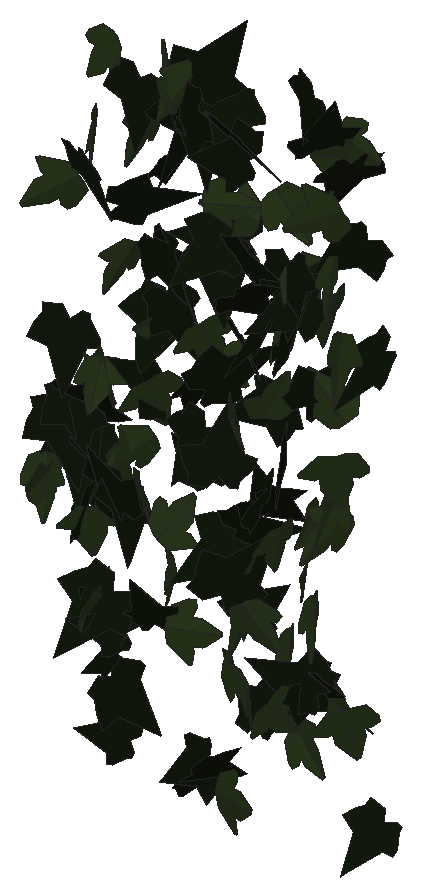
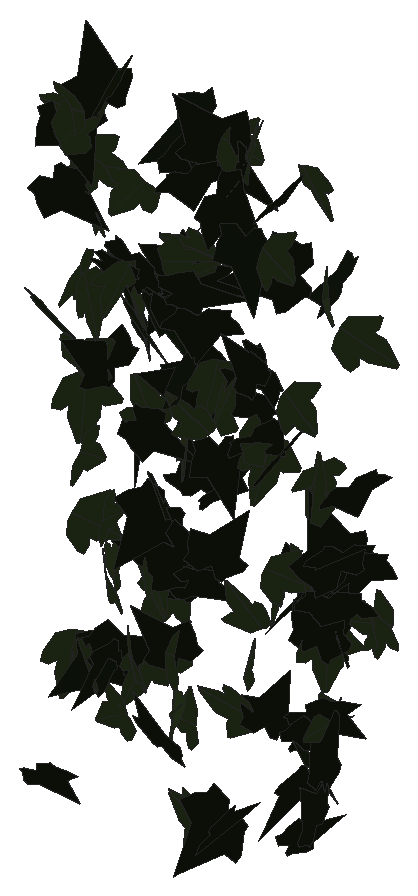
# SketchUp Ruby script. Lengths in inches.
U = 1.inch
M = Sketchup.active_model
def pt(a) = Geom::Point3d.new(a.map { |v| v * U })
def face(e, loops, mat)
  f = e.add_face(loops[0].map { |a| pt(a) })
  loops[1..].each { |l| e.add_face(l.map { |a| pt(a) }).erase! }
  f.material = f.back_material = mat if mat
  f
end
# faces: each face lists its corners as indices into pts; further lists are holes
def faces(e, pts, list, mat = nil) = list.each { |f| face(e, (f[0].is_a?(Array) ? f : [f]).map { |l| l.map { |i| pts[i] } }, mat) }
# xy, xz, yz: faces in a plane at the given z, y or x. An outline is a flat list of corners, or four numbers for a rectangle; further outlines are holes
def ring(l) = l.size == 4 ? [[l[0], l[1]], [l[2], l[1]], [l[2], l[3]], [l[0], l[3]]] : l.each_slice(2).to_a
def flat(e, list, mat, &to3) = list.each { |f| face(e, (f[0].is_a?(Array) ? f : [f]).map { |l| ring(l).map { |u, v| to3.(u, v) } }, mat) }
def xy(e, z, list, mat = nil) = flat(e, list, mat) { |x, y| [x, y, z] }
def xz(e, y, list, mat = nil) = flat(e, list, mat) { |x, z| [x, y, z] }
def yz(e, x, list, mat = nil) = flat(e, list, mat) { |y, z| [x, y, z] }
def lines(e, pts, list) = list.each { |a, b| e.add_line(pt(pts[a]), pt(pts[b])) }
# prism: a flat outline (further loops are holes) pulled along v
def prism(e, loops, v, mat = nil)
  f = face(e, loops, mat); d = Geom::Vector3d.new(v.map { |x| x * U })
  f.pushpull(f.normal.samedirection?(d) ? d.length : -d.length)
end
def box(e, o, s, mat = nil) = prism(e, [[o, [o[0] + s[0], o[1], o[2]], [o[0] + s[0], o[1] + s[1], o[2]], [o[0], o[1] + s[1], o[2]]]], [0, 0, s[2]], mat)
def at(x, y, z, deg = 0) = Geom::Transformation.translation(pt([x, y, z])) * Geom::Transformation.rotation(ORIGIN, Z_AXIS, deg.degrees)
def axes(o, x, y, z) = Geom::Transformation.new([*x, 0, *y, 0, *z, 0, *pt(o).to_a, 1])
def part(name) = M.definitions.add(name)
# library, detail: a bought-in or finely detailed component or shape, given as its bounding box
def library(name, o, s) = part(name).tap { |d| box(d.entities, o, s) }
def detail(e, o, s) = box(e.add_group.entities, o, s)
def put(e, d, t, mat = nil) = e.add_instance(d, t).tap { |i| i.material = mat if mat }
def group(e, t, mat = nil) = e.add_group.tap { |g| g.transformation = t; g.material = mat if mat }.entities
root = M.entities
M.materials.add("efeu1").color = [18, 25, 13]
M.materials.add("efeu2").color = [43, 57, 29]
c1 = part("ivyleaf_9")
p = [[1.54,2.16,1.25],[1.36,2.04,1.19],[-0.21,0.99,0.68],[-0.71,1.11,0.82],[-0.85,0.86,0.67],[-0.8,0.17,0.21],
  [-0.9,-0.01,0.1],[-0.67,-0.16,-0.02],[-0.08,-0.08,-0.05],[-0.03,-0.6,-0.4],[0.65,-0.88,-0.66],[0.83,-0.6,-0.49],
  [1.29,-0.42,-0.43],[1.8125,-0.07,-0.26],[1.21,0.44,0.15]]
faces(c1.entities,p,[[0,1,2,3,4,5,6,7,8,9,10,11,12,13,14]],"efeu1")
c2 = part("ivyleaf_10")
p = [[0,0.5,-0.03],[-0.0625,2.02,-0.43],[-0.19,2.01,-0.46],[-0.54,1.05,-0.29],[-0.52,0.625,-0.18],[-0.83,0.76,-0.28],
  [-1.16,0.64,-0.33],[-1.15,0.33,-0.24],[-0.77,-0.39,0.02],[-0.3,-0.51,0.16],[0.04,-0.48,0.23],[-0.02,2.01,-0.4375],
  [-0.06,2.01,-0.43],[0.04,-0.49,0.23],[0.67,-0.49,0.14],[1.38,0.36,-0.2],[1.375,0.51,-0.24],[0.81,0.65,-0.19],
  [0.62,0.59,-0.15],[0.6,1.09,-0.28],[0.5,1.23,-0.31]]
faces(c2.entities,p,[[0,1,2,3,4,5,6,7,8,9,10],[11,12,0,13,14,15,16,17,18,19,20]],"efeu2")
put(root,c1,axes([582.67,122.77,220.07],[0.28536,-0.15616,1.05734],[-0.80037,0.69407,0.31852],[-0.70835,-0.84714,0.06606]))
put(root,c1,axes([588.17,122.66,241.81],[1.27243,-0.37924,0.13675],[0.15917,0.05661,-1.32403],[0.37039,1.27851,0.09919]))
put(root,c2,axes([589.89,122.82,217.29],[-0.96033,-0.08304,-0.64359],[0.64471,0.00878,-0.96313],[0.07388,-1.15601,0.03892]))
put(root,c2,axes([581.11,123.12,226.61],[0.5179,0.83817,-0.30475],[-0.14661,-0.2676,-0.98515],[-0.87972,0.53804,-0.01523]))
put(root,c1,axes([588.96,123.8,239.69],[-0.18328,-0.19881,1.10316],[-0.78548,-0.77468,-0.27011],[0.79968,-0.80649,-0.01248]))
put(root,c1,axes([588.7,122.47,218.12],[-0.32325,-0.20959,1.28643],[1.2402,0.35822,0.37],[-0.40091,1.27713,0.10734]))
put(root,c1,axes([579.77,123.35,236.83],[0.6901,-0.88624,0.28676],[0.19189,-0.21397,-1.12307],[0.9115,0.71602,0.01933]))
put(root,c2,axes([591.46,122.6,213.15],[-0.35863,-0.88225,-0.74204],[0.32602,0.66778,-0.95152],[1.10576,-0.48303,0.03988]))
put(root,c2,axes([594.68,123.41,232.29],[-0.06394,1.06124,-0.60286],[0.0174,-0.60283,-1.06304],[-1.2204,-0.06419,0.01643]))
put(root,c2,axes([593.94,123.51,235.95],[0.82287,-0.508,0.51793],[0.42868,-0.29134,-0.96684],[0.58527,0.92762,-0.02003]))
put(root,c2,axes([577.73,123.36,220.26],[1.14299,-0.24618,0.39364],[0.38303,-0.09114,-1.16917],[0.26239,1.20543,-0.008]))
put(root,c1,axes([589.43,122.48,233.45],[0.69821,0.84288,0.17455],[0.08689,0.15459,-1.09406],[-0.85637,0.7029,0.03131]))
put(root,c1,axes([590.52,123.31,232.22],[-0.98424,0.71194,-0.38246],[0.29558,-0.24381,-1.21452],[-0.75217,-1.02741,0.02319]))
put(root,c1,axes([580.99,124.01,214.65],[-0.97786,-0.82422,0.26843],[-0.18701,-0.19454,-1.27858],[0.84641,-0.99519,0.02762]))
put(root,c2,axes([577.98,122.57,219.63],[0.18924,-0.52337,0.92037],[-0.11876,0.91856,0.54676],[-1.05209,-0.19783,0.10382]))
put(root,c1,axes([579.5,123.39,218.09],[-0.16511,0.70017,0.81678],[0.191,-0.79414,0.71937],[1.05872,0.25246,-0.0024]))
put(root,c2,axes([594.54,123.25,226.29],[-0.88855,-0.87624,-0.0737],[0.05581,0.04837,-1.24792],[0.87756,-0.89029,0.00474]))
put(root,c1,axes([582.89,122.56,235.84],[0.62541,0.27606,1.02935],[0.92812,0.44551,-0.68339],[-0.52379,1.11903,0.01813]))
put(root,c2,axes([584.07,123.14,226.61],[-0.60377,-0.98821,-0.40076],[0.21859,0.33607,-1.15801],[1.04374,-0.64203,0.01069]))
put(root,c1,axes([582.07,123.92,207.55],[-0.27991,0.0033,0.88175],[-0.73393,-0.51362,-0.23106],[0.48872,-0.76943,0.15803]))
put(root,c2,axes([585.36,124.14,242.44],[-0.19289,-0.69452,0.88742],[0.0379,-0.90382,-0.69911],[1.12625,-0.08853,0.17551]))
put(root,c2,axes([593.85,123.75,238.63],[-0.49289,-0.29297,1.13506],[-0.97891,-0.57454,-0.57338],[0.64492,-1.09599,-0.00284]))
put(root,c1,axes([591.26,123.22,230.83],[-0.35209,1.08034,0.65143],[0.15401,-0.63446,1.13543],[1.25211,0.38182,0.04352]))
put(root,c1,axes([583.64,124.07,225.92],[0.18255,-1.13857,-0.12958],[0.04306,-0.1243,1.15289],[-1.14511,-0.18619,0.0227]))
put(root,c1,axes([591.78,122.72,225.77],[0.02067,0.01104,-1.3144],[-1.19818,0.5407,-0.0143],[0.54049,1.19821,0.01856]))
put(root,c1,axes([581.8,123.98,212.98],[-0.34688,0.00817,0.88667],[-0.78351,-0.44862,-0.30239],[0.41517,-0.8398,0.17016]))
put(root,c1,axes([581.83,124.2,220.09],[0.18495,-1.24807,0.37799],[0.05148,-0.37449,-1.26169],[1.30303,0.19194,-0.0038]))
put(root,c2,axes([587.63,123.93,206.66],[0.11355,-0.06361,-1.21846],[0.98362,-0.71928,0.12922],[-0.72192,-0.99003,-0.01559]))
put(root,c1,axes([587.64,122.72,228.13],[0.18451,0.06574,1.31526],[1.16157,0.61763,-0.19382],[-0.62047,1.17579,0.02828]))
put(root,c1,axes([588.51,123.8,234.53],[0.4522,-0.3771,0.89753],[0.70614,-0.5542,-0.58862],[0.67017,0.83839,0.0146]))
put(root,c1,axes([587.83,123.23,223.51],[-0.97749,-0.16539,0.63639],[0.63888,0.03077,0.98931],[-0.15551,1.16599,0.06416]))
put(root,c1,axes([593.125,123.66,241.85],[0.82112,0.7523,0.49304],[-0.35711,-0.34005,1.11361],[0.82554,-0.89537,-0.00867]))
put(root,c2,axes([578.54,124.06,234.86],[-0.47611,-0.39925,1.03517],[-0.71009,-0.75588,-0.61812],[0.8525,-0.85259,0.06326]))
put(root,c1,axes([587.55,124.22,234.99],[-0.96818,-0.54092,0.3383],[-0.2777,-0.19624,-1.10851],[0.5744,-1.00663,0.03431]))
put(root,c1,axes([581.73,123.49,212.17],[-0.7287,0.61086,0.10739],[-0.08069,0.07091,-0.95087],[-0.61495,-0.73315,-0.00249]))
put(root,c1,axes([585.98,124.41,224.6],[-0.32402,-0.93712,0.43634],[-0.15865,-0.40677,-0.99143],[1.02147,-0.36044,-0.01557]))
put(root,c1,axes([586.2,123.625,241.32],[-0.17012,-0.01016,-1.25752],[-1.15516,-0.5003,0.16032],[-0.49705,1.16619,0.05782]))
put(root,c2,axes([593.72,124.28,223.72],[0.03279,0.69958,-0.9135],[-0.08101,-0.9102,-0.69996],[-1.14775,0.08423,0.0233]))
put(root,c2,axes([580.67,122.875,213.81],[0.16842,-0.09147,1.07306],[-0.32904,1.02979,0.13943],[-1.02545,-0.34546,0.1315]))
put(root,c2,axes([580.3,123.74,218.57],[-0.73455,-0.94584,-0.00263],[0.00648,-0.0017,-1.19755],[0.94582,-0.73456,0.00616]))
put(root,c1,axes([581.78,123.29,210.82],[0.45602,-0.6841,-0.98124],[-0.35387,0.92597,-0.81002],[1.14263,0.55979,0.14075]))
put(root,c1,axes([592.55,124.11,233.75],[-1.25015,0.09088,0.3312],[-0.33335,-0.02029,-1.25271],[-0.08262,-1.29311,0.04293]))
put(root,c1,axes([578.52,123.97,223.24],[-0.44564,-0.98323,-0.68623],[0.2876,0.62307,-1.0795],[1.16402,-0.53037,0.004]))
put(root,c2,axes([580.76,123.94,225.21],[-1.09801,0.50083,0.28511],[0.25705,-0.12347,1.20682],[0.51579,1.12768,0.0055]))
put(root,c1,axes([592.53,124.09,213.59],[-0.21715,0.03685,1.14232],[-1.14044,0.06941,-0.21904],[-0.0751,-1.1607,0.02317]))
put(root,c2,axes([594.78,123.69,213.2],[-0.80607,-0.88088,-0.24425],[0.16575,0.1794,-1.19403],[0.89897,-0.82293,0.00115]))
put(root,c1,axes([582.2,124.6,240.99],[0.02506,-1.20715,0.33415],[0.07808,-0.33206,-1.20546],[1.25011,0.04493,0.06859]))
put(root,c2,axes([584.91,123.42,241.58],[-0.52471,1.0044,-0.57786],[-0.26012,0.51606,1.13317],[1.12919,0.5856,-0.00748]))
put(root,c2,axes([592.23,124.34,217.6875],[0.78968,-0.48284,0.76635],[0.6527,-0.40159,-0.92559],[0.62802,1.0245,-0.00164]))
put(root,c1,axes([578.3,124.47,227.38],[-0.26941,-1.14556,-0.1084],[0.02543,0.10538,-1.17682],[1.1504,-0.27061,0.00063]))
put(root,c2,axes([588.17,124.65,211.875],[-0.4091,-0.12241,1.15089],[0.93463,-0.75491,0.25194],[0.68264,0.96022,0.34479]))
put(root,c2,axes([590.74,124.17,232.14],[0.77943,-0.99061,-0.05594],[-0.0321,0.04592,-1.26048],[0.99166,0.78009,0.00317]))
put(root,c1,axes([587.6875,124.69,219.34],[-1.00284,-0.47753,0.46517],[-0.40567,-0.22963,-1.11031],[0.529,-1.08136,0.03037]))
put(root,c1,axes([590.98,124.3,234.72],[-0.8277,-0.27917,-0.92575],[0.8756,0.30058,-0.8735],[0.41021,-1.20488,-0.00342]))
put(root,c2,axes([582.1,123.76,221.9],[-0.22941,0.17464,0.94755],[-0.93348,0.20101,-0.26305],[-0.23869,-0.95398,0.11804]))
put(root,c2,axes([591.58,124.21,210.96],[0.56503,-0.02066,0.98754],[0.98694,-0.03441,-0.56541],[0.04013,1.13724,0.00083]))
put(root,c2,axes([586.5,123.89,230.1],[-0.56279,-0.94475,-0.38083],[0.22119,0.31136,-1.09929],[0.99432,-0.604,0.02899]))
put(root,c1,axes([589.99,123.48,222.55],[-0.67867,0.29001,-0.80103],[-0.75256,0.27587,0.73748],[0.39925,1.01298,0.02849]))
put(root,c2,axes([590.84,123.9375,238.2],[0.77992,0.36089,0.74312],[0.6499,0.36287,-0.85831],[-0.50999,1.01432,0.04266]))
put(root,c1,axes([585.65,125.13,207.28],[0.29523,-0.65632,-0.84207],[0.325,-0.77696,0.71952],[-1.01696,-0.43883,-0.01452]))
put(root,c2,axes([588.36,123.58,226.39],[-0.52993,0.4216,0.99529],[-0.73927,0.66731,-0.67628],[-0.78856,-0.90892,-0.03485]))
put(root,c2,axes([593.81,124.3,228.3],[0.82273,0.29156,0.77588],[-0.72186,-0.28519,0.87262],[0.40732,-1.09432,-0.02069]))
put(root,c2,axes([583.8,124.89,216.21],[-0.15956,0.1299,1.02445],[0.7048,-0.74393,0.2041],[0.75474,0.72216,0.02599]))
put(root,c2,axes([580.68,124.31,242.49],[0.91701,-0.40513,-0.42947],[-0.40344,0.14927,-1.00222],[0.43107,1.00154,-0.02436]))
put(root,c2,axes([590.38,124.33,220.82],[-0.07661,-1.06379,-0.08029],[0.01751,0.07924,-1.06648],[1.06668,-0.07771,0.01174]))
put(root,c1,axes([595.05,124.625,237.32],[0.10016,0.18581,-1.08768],[-0.62083,-0.8934,-0.20979],[-0.91222,0.62843,0.02335]))
put(root,c1,axes([591.65,125.18,243.12],[0.04195,-0.81298,0.81091],[0.11823,-0.80408,-0.81225],[1.14216,0.11309,0.05429]))
put(root,c2,axes([582.57,124.12,220.71],[-0.7221,0.6444,0.13979],[-0.09997,0.09792,-0.9678],[-0.65177,-0.72895,-0.00643]))
put(root,c1,axes([583.03,124.625,213.63],[0.66027,-0.05796,0.65623],[-0.6521,0.07446,0.66269],[-0.09357,-0.92792,0.01219]))
put(root,c1,axes([580.04,124.64,218.88],[0.85334,-0.41988,0.80531],[-0.70123,0.39762,0.95037],[-0.57715,-1.10391,0.03601]))
put(root,c2,axes([589.79,124.37,226.96],[-0.49668,-0.90904,0.28806],[0.14676,0.24806,1.03583],[-0.94223,0.51782,0.00949]))
put(root,c2,axes([587.84,125.21,215.71],[0.12947,-0.64646,1.039],[0.52958,-0.9123,-0.63361],[1.10317,0.51382,0.18223]))
put(root,c1,axes([578.68,124.57,223.86],[-0.24171,-0.94463,-0.66097],[0.21609,0.62625,-0.97403],[1.13248,-0.32111,0.04478]))
put(root,c1,axes([579.375,125.1,212.48],[0.14201,0.38621,1.16865],[-0.39302,-1.10058,0.41147],[1.16637,-0.41788,-0.00364]))
put(root,c1,axes([578.74,124.73,223.21],[1.28625,0.26152,-0.16077],[0.15574,0.0409,1.31254],[0.26454,-1.29561,0.00898]))
put(root,c1,axes([585.3,125.18,239.71],[0.24538,-1.12581,0.37947],[0.0798,-0.37099,-1.15224],[1.18536,0.25803,-0.00098]))
put(root,c1,axes([587.51,125.08,229.67],[0.39981,-0.69204,0.72907],[0.35865,-0.63477,-0.79921],[0.93906,0.53708,-0.00516]))
put(root,c2,axes([586.68,124.44,236.42],[0.16254,-0.09909,-1.10519],[1.1084,-0.03787,0.16641],[-0.05202,-1.11643,0.09245]))
put(root,c2,axes([589.37,124.78,219.57],[0.28854,-1.20887,0.08828],[0.01684,-0.08674,-1.24282],[1.21197,0.28901,-0.00375]))
put(root,c1,axes([592.38,123.92,228.41],[-0.1532,-0.07308,1.12984],[0.96449,0.58873,0.16886],[-0.593,0.97643,-0.01726]))
put(root,c2,axes([593.6875,125.43,240.64],[-0.23209,-0.41819,-1.13662],[-0.51861,-1.01152,0.47806],[-1.09446,0.56799,0.01451]))
put(root,c1,axes([594.41,124.47,241.04],[0.05048,1.02371,-0.61251],[-0.09344,-0.60778,-1.02351],[-1.18929,0.09121,0.05442]))
put(root,c1,axes([583.73,124.76,230.48],[-0.26049,-0.3477,-1.1571],[1.05438,0.51257,-0.39138],[0.58996,-1.06958,0.18859]))
put(root,c1,axes([579,125.04,221.57],[-0.77966,-0.90702,-0.51552],[0.35948,0.37061,-1.19572],[0.9794,-0.85807,0.02849]))
put(root,c2,axes([584.34,124.71,213.77],[0.16746,-0.20437,-1.17963],[1.1645,-0.24872,0.2084],[-0.27794,-1.16521,0.16242]))
put(root,c2,axes([591.17,125.37,218.92],[-0.03298,-0.33621,-0.99543],[0.28908,-0.96038,0.3148],[-1.01012,-0.26387,0.12259]))
put(root,c2,axes([586.94,124.98,212.45],[0.20835,-0.25214,1.07146],[1.06478,-0.23024,-0.26123],[0.27901,1.06697,0.19683]))
put(root,c1,axes([585.12,125.36,240.35],[-0.27086,0.44863,-1.26807],[0.68634,-1.06637,-0.52387],[-1.15681,-0.73772,-0.0139]))
put(root,c2,axes([583.8,124.5,218.66],[0.92933,-0.00345,-0.60627],[0.60548,0.06219,0.92777],[0.03109,-1.10786,0.05397]))
put(root,c2,axes([581.87,125.36,222.08],[-0.2279,-0.46669,0.92718],[-0.29107,-0.88245,-0.51572],[0.99636,-0.36454,0.06142]))
put(root,c1,axes([586.08,123.73,207.29],[0.60187,0.96743,0.61569],[0.28172,0.54929,-1.13849],[-1.11159,0.66303,0.04483]))
put(root,c1,axes([592.01,124.1,213.83],[0.1838,-0.2267,-1.04176],[-0.37842,0.97442,-0.27881],[0.99672,0.41176,0.08625]))
put(root,c2,axes([590.09,125.3,214.83],[0.78406,-0.52836,0.80453],[0.659,-0.46164,-0.94541],[0.70154,1.02416,-0.01108]))
put(root,c2,axes([587.9375,125.12,235.85],[0.19231,0.1832,1.06547],[-0.88572,-0.59383,0.26197],[0.6199,-0.9053,0.04378]))
put(root,c2,axes([593.95,124.33,213.04],[0.21242,-0.21413,-1.11299],[-0.79921,0.77463,-0.30157],[0.80366,0.82694,-0.00571]))
put(root,c2,axes([591.51,125.48,221.64],[-0.00955,0.36078,-0.96223],[0.00377,-0.96225,-0.36082],[-1.02763,-0.00688,0.00762]))
put(root,c1,axes([585.82,124.43,242.12],[-0.53882,-0.17609,1.14757],[1.14165,0.14966,0.559],[-0.21108,1.2589,0.09406]))
put(root,c1,axes([587.91,124.625,220.07],[0.45446,-0.09746,1.03287],[1.02879,-0.10314,-0.4624],[0.13385,1.12371,0.04714]))
put(root,c1,axes([592.37,124.6,213.76],[1.13399,-0.14508,0.1181],[0.11742,-0.01282,-1.14323],[0.14563,1.14005,0.00217]))
put(root,c2,axes([578.85,125.49,237.26],[0.34014,-0.2863,0.97578],[0.74357,-0.63187,-0.44459],[0.6937,0.81767,-0.00191]))
put(root,c1,axes([589.88,125.16,226.93],[-0.1463,-0.04731,-1.12376],[-0.82799,-0.76247,0.1399],[-0.76126,0.83839,0.06381]))
put(root,c1,axes([589.38,124.16,222.24],[0.80356,0.83731,0.26818],[0.16951,0.20896,-1.16031],[-0.86271,0.82095,0.02181]))
put(root,c1,axes([587.625,125.31,234.47],[-0.70894,0.01881,0.95009],[-0.94922,-0.06991,-0.7069],[0.04481,-1.18337,0.05687]))
put(root,c2,axes([583.0625,125.67,228.45],[-0.1423,-0.12341,-0.98622],[-0.44068,-0.88516,0.17435],[-0.89088,0.45756,0.07128]))
put(root,c1,axes([584.25,124.53,238.04],[-0.11494,1.19731,-0.10819],[0.00949,-0.10778,-1.20282],[-1.20215,-0.11533,0.00085]))
put(root,c1,axes([586.36,125.27,233.625],[-0.60264,-0.91496,-0.60108],[0.32802,0.5037,-1.09559],[1.04444,-0.68612,-0.00274]))
put(root,c1,axes([595.34,125.47,207.23],[-0.90634,-0.44663,0.02255],[-0.01936,-0.01173,-1.01041],[0.44677,-0.90654,0.00196]))
put(root,c2,axes([581.94,125.64,238.53],[-0.01381,-0.90295,0.70048],[0.12409,-0.69757,-0.89676],[1.13605,0.06522,0.10647]))
put(root,c1,axes([595.39,125.44,231.29],[-1.15301,0.17909,-0.33272],[0.29228,-0.2544,-1.14981],[-0.23947,-1.17278,0.19861]))
put(root,c2,axes([580.79,125.54,231.39],[-0.10431,-0.92547,0.56781],[-0.05392,-0.56531,-0.9313],[1.08444,-0.11713,0.00831]))
put(root,c1,axes([587.91,124.94,215.57],[-0.18186,-0.06894,1.01165],[0.97996,-0.27601,0.15735],[0.26052,0.99012,0.11431]))
put(root,c2,axes([593.57,125.26,241.79],[-0.21572,-0.05911,-1.08823],[1.00129,-0.44876,-0.17411],[-0.43031,-1.01459,0.14041]))
put(root,c1,axes([585.54,124.84,226.93],[-0.07399,1.01548,-0.36408],[0.02819,-0.36299,-1.01817],[-1.0784,-0.07916,-0.00164]))
put(root,c2,axes([585.24,125,228.89],[-0.84636,0.58733,-0.29935],[-0.24983,0.16504,1.03016],[0.61004,0.88244,0.00657]))
put(root,c1,axes([579.27,125.79,210.32],[0.29754,-0.59523,0.94998],[0.3825,-0.86999,-0.66491],[1.05378,0.48385,-0.02689]))
put(root,c1,axes([582.73,125.87,229.07],[-0.56157,-1.07736,0.16593],[-0.05954,-0.15606,-1.21479],[1.08844,-0.5644,0.01916]))
put(root,c1,axes([588.94,124.74,210.6],[-0.87916,0.64297,0.5186],[0.40007,-0.33117,1.08883],[0.7227,0.9655,0.02812]))
put(root,c2,axes([592.46,125.95,221.46],[-0.19564,-0.67296,1.01536],[-0.04143,-1.02411,-0.68673],[1.21742,-0.143,0.1398]))
put(root,c2,axes([586.52,124.95,227.85],[0.71753,0.02191,-0.77898],[0.77614,0.07501,0.71703],[0.06999,-1.05643,0.03476]))
put(root,c2,axes([592.63,125.31,233.04],[0.13496,-1.23518,-0.02098],[0.00013,0.02112,-1.24253],[1.23535,0.13494,0.00242]))
put(root,c1,axes([585.39,125.47,221.43],[0.55621,-0.03355,0.8539],[-0.85358,0.02707,0.55706],[-0.041,-1.01871,-0.01332]))
put(root,c1,axes([582.48,125.36,232.48],[-0.12503,-0.20114,-1.0869],[1.04157,0.34473,-0.18361],[0.37003,-1.03833,0.14959]))
put(root,c1,axes([582.98,125.5,231.67],[0.10261,-0.11628,0.98708],[0.69734,-0.69867,-0.15479],[0.70822,0.70478,0.0094]))
put(root,c2,axes([591.03,124.8,234.16],[0.13112,1.12412,0.39688],[0.0579,0.3928,-1.13169],[-1.19072,0.14289,-0.01133]))
put(root,c1,axes([590.13,125.49,232.79],[-0.9755,0.33031,-0.36441],[0.33582,-0.14406,-1.02955],[-0.35934,-1.03133,0.0271]))
put(root,c1,axes([586.6,125.71,241.09],[-0.40983,-1.09276,-0.27634],[0.10122,0.25717,-1.16707],[1.1226,-0.42212,0.00435]))
